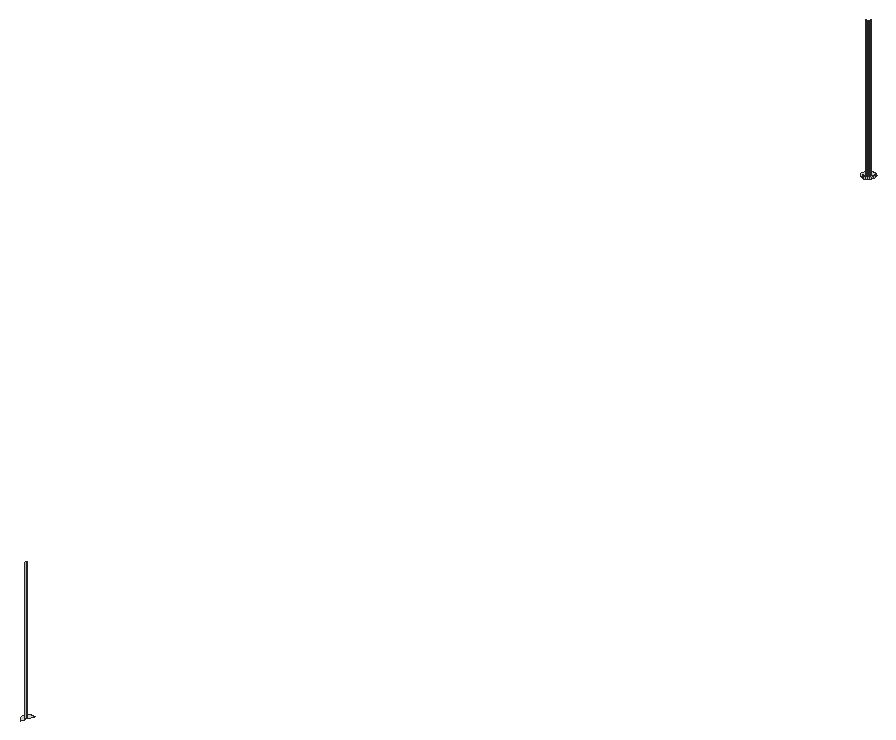
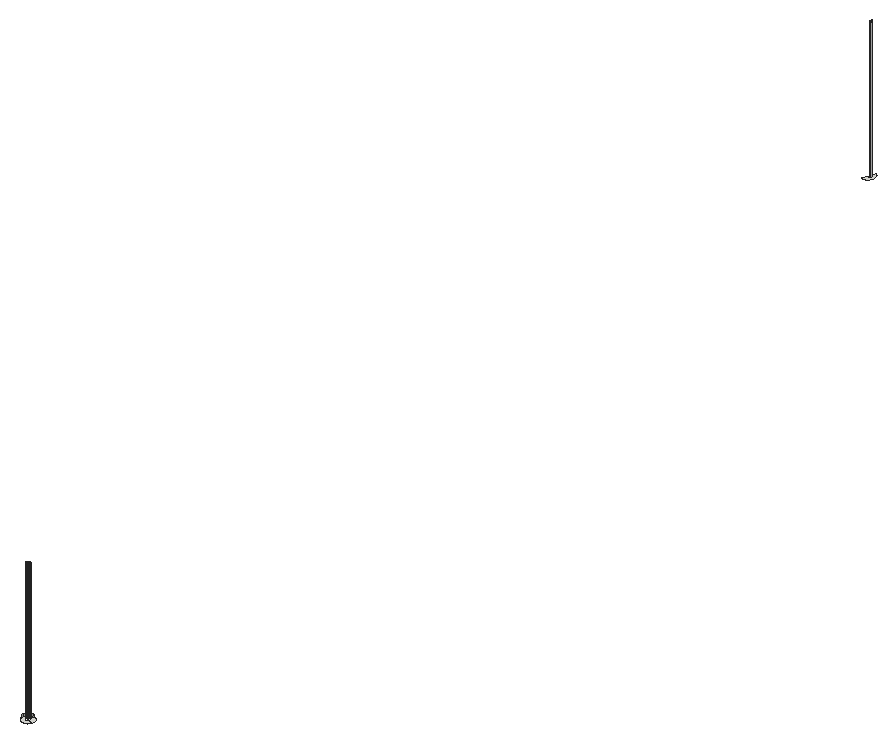
# SketchUp Ruby script. Lengths in inches.
U = 1.inch
M = Sketchup.active_model
def pt(a) = Geom::Point3d.new(a.map { |v| v * U })
def face(e, loops, mat)
  f = e.add_face(loops[0].map { |a| pt(a) })
  loops[1..].each { |l| e.add_face(l.map { |a| pt(a) }).erase! }
  f.material = f.back_material = mat if mat
  f
end
# faces: each face lists its corners as indices into pts; further lists are holes
def faces(e, pts, list, mat = nil) = list.each { |f| face(e, (f[0].is_a?(Array) ? f : [f]).map { |l| l.map { |i| pts[i] } }, mat) }
# xy, xz, yz: faces in a plane at the given z, y or x. An outline is a flat list of corners, or four numbers for a rectangle; further outlines are holes
def ring(l) = l.size == 4 ? [[l[0], l[1]], [l[2], l[1]], [l[2], l[3]], [l[0], l[3]]] : l.each_slice(2).to_a
def flat(e, list, mat, &to3) = list.each { |f| face(e, (f[0].is_a?(Array) ? f : [f]).map { |l| ring(l).map { |u, v| to3.(u, v) } }, mat) }
def xy(e, z, list, mat = nil) = flat(e, list, mat) { |x, y| [x, y, z] }
def xz(e, y, list, mat = nil) = flat(e, list, mat) { |x, z| [x, y, z] }
def yz(e, x, list, mat = nil) = flat(e, list, mat) { |y, z| [x, y, z] }
def lines(e, pts, list) = list.each { |a, b| e.add_line(pt(pts[a]), pt(pts[b])) }
# prism: a flat outline (further loops are holes) pulled along v
def prism(e, loops, v, mat = nil)
  f = face(e, loops, mat); d = Geom::Vector3d.new(v.map { |x| x * U })
  f.pushpull(f.normal.samedirection?(d) ? d.length : -d.length)
end
def box(e, o, s, mat = nil) = prism(e, [[o, [o[0] + s[0], o[1], o[2]], [o[0] + s[0], o[1] + s[1], o[2]], [o[0], o[1] + s[1], o[2]]]], [0, 0, s[2]], mat)
def at(x, y, z, deg = 0) = Geom::Transformation.translation(pt([x, y, z])) * Geom::Transformation.rotation(ORIGIN, Z_AXIS, deg.degrees)
def axes(o, x, y, z) = Geom::Transformation.new([*x, 0, *y, 0, *z, 0, *pt(o).to_a, 1])
def part(name) = M.definitions.add(name)
# library, detail: a bought-in or finely detailed component or shape, given as its bounding box
def library(name, o, s) = part(name).tap { |d| box(d.entities, o, s) }
def detail(e, o, s) = box(e.add_group.entities, o, s)
def put(e, d, t, mat = nil) = e.add_instance(d, t).tap { |i| i.material = mat if mat }
def group(e, t, mat = nil) = e.add_group.tap { |g| g.transformation = t; g.material = mat if mat }.entities
root = M.entities
M.materials.add("[Color_000]").color = [255, 255, 255]
xy(root,321.27,[[944.63,768.75,945.01,769.62,944.92,769.68,944.8125,769.8,944.74,769.95,944.71,770.11,944.72,770.27,944.77,770.43,944.86,770.57,944.98,770.68,945.13,770.75,945.29,770.78,945.45,770.77,945.51,770.76,945.88,771.62,945.63,771.7,945.22,771.73,944.82,771.64,944.45,771.46,944.14,771.19,943.92,770.84,943.79,770.45,943.76,770.04,943.85,769.64,944.03,769.27,944.3,768.96],[938.05,1048.34,937.64,1048.37,937.25,1048.5,936.91,1048.72,936.64,1049.03,936.45,1049.4,936.37,1049.8,936.4,1050.21,936.5,1050.54,937.37,1050.17,937.32,1050.03,937.3125,1049.87,937.35,1049.71,937.42,1049.5625,937.53,1049.4375,937.67,1049.35,937.82,1049.3,937.99,1049.29,938.15,1049.32,938.29,1049.39,938.42,1049.5,938.51,1049.64,938.52,1049.66,939.38,1049.29,939.36,1049.23,939.13,1048.88,938.82,1048.61,938.46,1048.43],[[938.05,1048.34,937.64,1048.37,937.25,1048.5,936.91,1048.72,936.64,1049.03,936.45,1049.4,936.37,1049.8,936.4,1050.21,936.5,1050.54,936.52,1050.6,936.75,1050.95,937.06,1051.22,937.43,1051.4,937.83,1051.49,938.24,1051.46,938.63,1051.33,938.97,1051.11,939.25,1050.8,939.43,1050.43,939.51,1050.03,939.49,1049.62,939.36,1049.23,939.13,1048.88,938.82,1048.61,938.46,1048.43],[937.99,1049.29,938.15,1049.32,938.29,1049.39,938.42,1049.5,938.51,1049.64,938.52,1049.66,938.56,1049.8,938.57,1049.96,938.54,1050.12,938.46,1050.27,938.35,1050.39,938.22,1050.48,938.0625,1050.53,937.9,1050.54,937.74,1050.51,937.59,1050.4375,937.47,1050.33,937.375,1050.19,937.37,1050.17,937.32,1050.03,937.3125,1049.87,937.35,1049.71,937.42,1049.5625,937.53,1049.4375,937.67,1049.35,937.82,1049.3]]])
xy(root,321.27,[[937.99,1049.29,937.82,1049.3,937.67,1049.35,937.53,1049.4375,937.42,1049.5625,937.35,1049.71,937.3125,1049.87,937.32,1050.03,937.37,1050.17,938.52,1049.66,938.51,1049.64,938.42,1049.5,938.29,1049.39,938.15,1049.32]],"[Color_000]")
p = [[944.71,770.11,321.27],[944.74,769.95,321.27],[944.74,769.95,357.27],[944.71,770.11,357.27],[944.72,770.27,321.27],[944.72,770.27,357.27],
  [944.77,770.43,321.27],[944.77,770.43,357.27],[937.64,1048.37,321.27],[938.05,1048.34,321.27],[938.05,1048.34,321.86],[937.64,1048.37,321.86],
  [938.46,1048.43,321.27],[938.46,1048.43,321.86],[938.82,1048.61,321.27],[938.82,1048.61,321.86],[939.13,1048.88,321.27],[939.13,1048.88,321.86],
  [939.36,1049.23,321.27],[939.36,1049.23,321.86],[939.38,1049.29,321.27],[939.49,1049.62,321.27],[939.49,1049.62,321.86],[937.82,1049.3,321.27],
  [937.99,1049.29,321.27],[937.99,1049.29,357.27],[937.82,1049.3,357.27],[938.15,1049.32,321.27],[938.15,1049.32,357.27],[938.29,1049.39,321.27],
  [938.29,1049.39,357.27],[938.42,1049.5,321.27],[938.42,1049.5,357.27],[938.51,1049.64,321.27],[938.51,1049.64,357.27],[938.52,1049.66,321.27],
  [938.56,1049.8,321.27],[938.56,1049.8,357.27],[939.51,1050.03,321.27],[939.51,1050.03,321.86],[938.57,1049.96,321.27],[938.57,1049.96,357.27]]
faces(root,p,[[0,1,2,3],[4,0,3,5],[6,4,5,7],[23,24,25,26],[24,27,28,25],[27,29,30,28],[29,31,32,30],[31,33,34,32],
  [33,35,36,37,34],[36,40,41,37]],"[Color_000]")
faces(root,p,[[8,9,10,11],[9,12,13,10],[12,14,15,13],[14,16,17,15],[16,18,19,17],[18,20,21,22,19],[21,38,39,22]])
